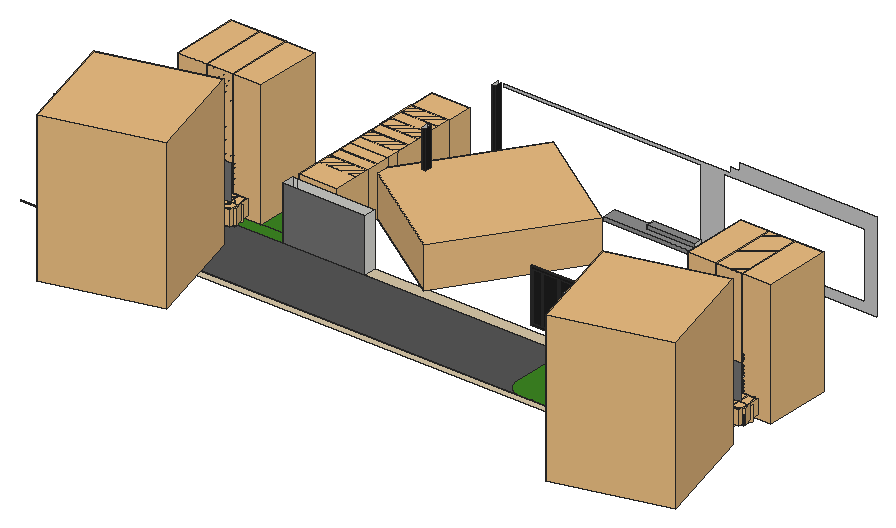
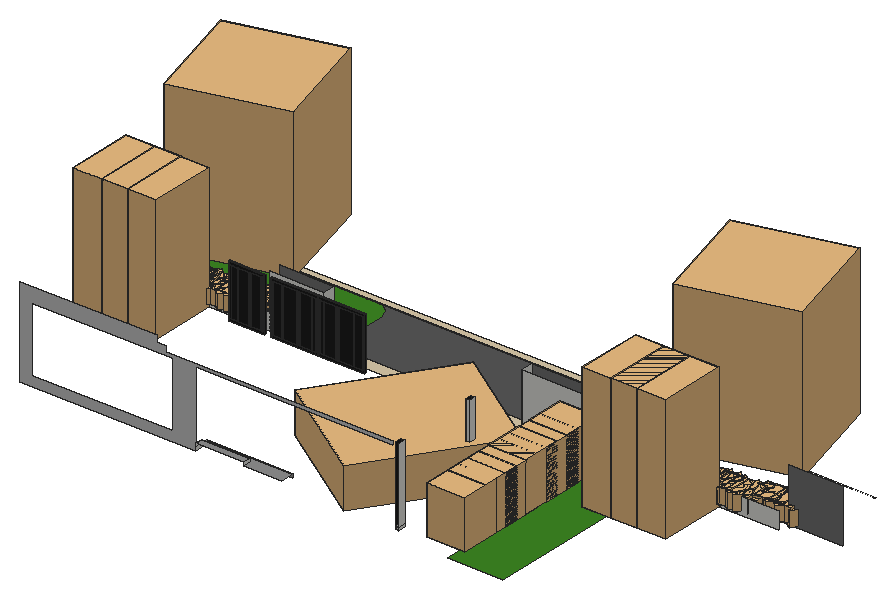
# SketchUp Ruby script. Lengths in inches.
U = 1.inch
M = Sketchup.active_model
def pt(a) = Geom::Point3d.new(a.map { |v| v * U })
def face(e, loops, mat)
  f = e.add_face(loops[0].map { |a| pt(a) })
  loops[1..].each { |l| e.add_face(l.map { |a| pt(a) }).erase! }
  f.material = f.back_material = mat if mat
  f
end
# faces: each face lists its corners as indices into pts; further lists are holes
def faces(e, pts, list, mat = nil) = list.each { |f| face(e, (f[0].is_a?(Array) ? f : [f]).map { |l| l.map { |i| pts[i] } }, mat) }
# xy, xz, yz: faces in a plane at the given z, y or x. An outline is a flat list of corners, or four numbers for a rectangle; further outlines are holes
def ring(l) = l.size == 4 ? [[l[0], l[1]], [l[2], l[1]], [l[2], l[3]], [l[0], l[3]]] : l.each_slice(2).to_a
def flat(e, list, mat, &to3) = list.each { |f| face(e, (f[0].is_a?(Array) ? f : [f]).map { |l| ring(l).map { |u, v| to3.(u, v) } }, mat) }
def xy(e, z, list, mat = nil) = flat(e, list, mat) { |x, y| [x, y, z] }
def xz(e, y, list, mat = nil) = flat(e, list, mat) { |x, z| [x, y, z] }
def yz(e, x, list, mat = nil) = flat(e, list, mat) { |y, z| [x, y, z] }
def lines(e, pts, list) = list.each { |a, b| e.add_line(pt(pts[a]), pt(pts[b])) }
# prism: a flat outline (further loops are holes) pulled along v
def prism(e, loops, v, mat = nil)
  f = face(e, loops, mat); d = Geom::Vector3d.new(v.map { |x| x * U })
  f.pushpull(f.normal.samedirection?(d) ? d.length : -d.length)
end
def box(e, o, s, mat = nil) = prism(e, [[o, [o[0] + s[0], o[1], o[2]], [o[0] + s[0], o[1] + s[1], o[2]], [o[0], o[1] + s[1], o[2]]]], [0, 0, s[2]], mat)
def at(x, y, z, deg = 0) = Geom::Transformation.translation(pt([x, y, z])) * Geom::Transformation.rotation(ORIGIN, Z_AXIS, deg.degrees)
def axes(o, x, y, z) = Geom::Transformation.new([*x, 0, *y, 0, *z, 0, *pt(o).to_a, 1])
def part(name) = M.definitions.add(name)
# library, detail: a bought-in or finely detailed component or shape, given as its bounding box
def library(name, o, s) = part(name).tap { |d| box(d.entities, o, s) }
def detail(e, o, s) = box(e.add_group.entities, o, s)
def put(e, d, t, mat = nil) = e.add_instance(d, t).tap { |i| i.material = mat if mat }
def group(e, t, mat = nil) = e.add_group.tap { |g| g.transformation = t; g.material = mat if mat }.entities
root = M.entities
M.materials.add("[Color M02]").color = [198, 198, 198]
M.materials.add("[Color M04]").color = [60, 133, 34]
M.materials.add("[Color M04]1").color = [142, 142, 142]
M.materials.add("[Color M05]1").color = [114, 114, 114]
M.materials.add("[Color M08]").color = [30, 30, 30]
M.materials.add("[Color_F16]").color = [51, 102, 0]
M.materials.add("[Field Square Tile]").color = [217, 201, 169]
M.materials.add("[Slate Light Tile]").color = [86, 86, 86]
c1 = library("Obj_000004",[-25.54,-25.36,-14.31],[50.67,50.64,41.42])
c2 = library("Obj_000003",[-31,-31.06,-7.89],[62,62.12,39.58])
c3 = library("Potted plant",[-29.7,0,-10.87],[31.67,38.52,72.45])
c4 = library("Palm tree",[-4.09,-4.52,0],[193.52,193.51,258.93])
c5 = part("Palm+Tree")
put(c5.entities,c4,at(25.51,-21.81,0,15))
c6 = library("plant (1)",[-35.72,-28.42,0],[66.31,67.39,84.38])
c7 = library("002+Bmw+M4+++mat3.4+2017",[-252.8,19.48,9.01],[196.94,171.32,55.15])
c8 = part("Group\#102")
g1 = group(c8.entities,at(0,0,0))
prism(g1,[[[0,3,72],[70.5,3,72],[70.5,3,0],[0,3,0]],[[67.5,3,3],[67.5,3,69],[3,3,69],[3,3,3]]],[0,-3,0])
c9 = part("Group\#135")
box(c9.entities,[0,0,0],[0.5,1,66])
c10 = part("Group\#148")
box(c10.entities,[0,-1,0],[5.5,1,66])
box(c10.entities,[50.84,-1,0],[13.66,1,66])
box(c10.entities,[28.06,-1,0],[22.28,1,66])
box(c10.entities,[24.66,-1,0],[2.9,1,66])
box(c10.entities,[6,-1,0],[18.16,1,66])
c11 = part("Component\#23")
g2 = group(c11.entities,at(70.5,0,0),"[Color M08]")
put(g2,c8,axes([70.5,0,0],[-1,0,0],[0,1,0],[0,0,1]))
g3 = group(g2,at(3,2,3))
g4 = group(g3,at(0,-1,0))
box(g4,[0,0,0],[5.5,1,66])
box(g4,[50.84,0,0],[13.66,1,66])
box(g4,[28.06,0,0],[22.28,1,66])
box(g4,[24.66,0,0],[2.9,1,66])
box(g4,[6,0,0],[18.16,1,66])
put(g3,c9,axes([50.34,0,0],[1,0,0],[0,-1,0],[0,0,1]))
put(g3,c9,axes([24.16,0,0],[1,0,0],[0,-1,0],[0,0,1]))
put(g3,c9,axes([27.56,0,0],[1,0,0],[0,-1,0],[0,0,1]))
put(g3,c9,axes([5.5,0,0],[1,0,0],[0,-1,0],[0,0,1]))
g5 = group(c11.entities,at(70.5,0,0),"[Color M08]")
put(g5,c8,at(-70.5,0,0))
g6 = group(g5,at(-3,2,3,-180))
put(g6,c10,at(0,1,0))
put(g6,c9,at(50.34,0,0))
put(g6,c9,at(24.16,0,0))
put(g6,c9,at(27.56,0,0))
put(g6,c9,at(5.5,0,0))
g7 = group(c11.entities,at(150,0,0),"[Color M08]")
put(g7,c8,axes([54,0,0],[-0.76596,0,0],[0,1,0],[0,0,1]))
g8 = group(g7,at(2.3,2,3))
put(g8,c10,axes([0,-1,0],[0.76596,0,0],[0,-1,0],[0,0,1]))
put(g8,c9,axes([38.55,0,0],[0.76596,0,0],[0,-1,0],[0,0,1]))
put(g8,c9,axes([18.5,0,0],[0.76596,0,0],[0,-1,0],[0,0,1]))
put(g8,c9,axes([21.11,0,0],[0.76596,0,0],[0,-1,0],[0,0,1]))
put(g8,c9,axes([4.22,0,0],[0.76596,0,0],[0,-1,0],[0,0,1]))
xy(root,-19.75,[[2463.16,10.6,2468.26,11.14,2473.25,12.39,2450.82,12.39,2452.96,11.68,2458.02,10.78],[1636.34,12.09,1641.55,12.39,1629.85,12.39,1631.12,12.24],[2522.8,12.09,2528.01,12.39,2516.3125,12.39,2517.58,12.24],[1938.63,143.39,1946.07,164.82],[1946.07,143.39,2081.32,164.82],
  [2037.07,322.71,2043.8,334.4375],[2037.07,475.3125,2043.8,487.3125]])
xy(root,-19.75,[[1841.83,12.39,1848.92,143.39],[2450.82,12.39,2735.38,12.39,2735.38,143.39,2426.02,143.39,2426.02,39.89,2427.39,34.93,2429.45,30.23,2432.14,25.85,2435.42,21.9,2439.22,18.4375,2443.47,15.55,2448.08,13.28],[1841.83,143.39,1938.63,164.82],[1841.83,164.82,1938.63,505.3125]],"[Color M04]")
xy(root,-19.75,[[2081.32,143.39,2426.02,164.82]],"[Field Square Tile]")
xy(root,-19.75,[[1848.92,12.39,2450.82,12.39,2448.08,13.28,2443.47,15.55,2439.22,18.4375,2435.42,21.9,2432.14,25.85,2429.45,30.23,2427.39,34.93,2426.02,39.89,2426.02,143.39,1848.92,143.39]],"[Slate Light Tile]")
xy(root,-19.3125,[[1841.83,0,1848.92,12.39],[1848.92,0,2735.38,12.39]],"[Field Square Tile]")
xy(root,-14.01,[[2240.94,464.0625,2391.36,464.0625,2391.36,474.5625,2306.98,474.5625,2306.98,487.3125,2240.94,487.3125]],"[Color M04]1")
xy(root,-8.01,[[2306.98,474.5625,2391.36,487.3125]],"[Color M04]1")
xz(root,12.39,[[1586.78,-19.75,1841.83,-19.3125],[1841.83,-19.75,1848.92,-19.3125],[1848.92,-19.75,2473.25,-19.3125],[2473.25,-19.75,2735.38,-19.3125]])
xz(root,143.39,[[1539.55,-19.75,1848.92,-19.75,1848.92,73,1787.65,73,1787.65,9.9375,1634.02,9.9375,1634.02,73,1539.55,73],[1938.63,-19.75,2081.32,73],[2426.02,-19.75,2735.38,-19.75,2735.38,73,2674.11,73,2674.11,9.9375,2520.48,9.9375,2520.48,73,2426.02,73]],"[Color M05]1")
xz(root,164.82,[[1634.02,-19.75,1787.65,9.9375],[1787.65,-19.75,1838.4,73],[1938.63,-19.75,1946.07,73],[1946.07,-19.75,1946.07,73,2081.32,73,2081.32,-19.75,2047.51,-19.75,2047.51,-15.625,2033.69,-15.625,2033.69,-19.75],[2033.69,-19.75,2047.51,-15.625],
  [2426.02,-19.75,2520.48,73],[2520.48,-19.75,2674.11,9.9375],[2674.11,-19.75,2724.86,73]])
xz(root,322.71,[[2037.07,-19.75,2043.8,-15.625]])
xz(root,322.71,[[2037.07,-15.625,2043.8,115.91]],"[Color M08]")
xz(root,334.4375,[[2037.07,-19.75,2043.8,-15.625],[2037.07,-15.625,2043.8,115.91]])
xz(root,464.0625,[[2240.94,-19.75,2391.36,-14.01]],"[Color M04]1")
xz(root,474.5625,[[2306.98,-14.01,2391.36,-8.01]],"[Color M04]1")
xz(root,475.3125,[[2037.07,-19.75,2043.8,-15.625]])
xz(root,475.3125,[[2037.07,-15.625,2043.8,115.91]],"[Color M08]")
xz(root,487.3125,[[2037.07,-19.75,2043.8,-15.625]])
xz(root,487.3125,[[[2391.36,-19.75,2696.7,-19.75,2696.7,136.125,2459.77,136.125,2459.77,125.0625,2444.15,125.0625,2444.15,123.92,2443.83,123.92,2443.83,117.06,2444.15,117.06,2444.15,115.91,2048.29,115.91,2048.29,110.1875,2391.36,110.1875],[2431.15,-3.75,2676.91,110.1875]]],"[Color M02]")
yz(root,1938.63,[[143.39,-19.75,164.82,73]])
yz(root,2037.07,[[322.71,-19.75,334.4375,-15.625],[475.3125,-19.75,487.3125,-15.625],[322.71,-15.625,334.4375,115.66],[475.3125,-15.625,487.3125,115.66]])
yz(root,2043.8,[[322.71,-19.75,334.4375,-15.625],[475.3125,-19.75,487.3125,-15.625]])
yz(root,2043.8,[[322.71,-15.625,334.4375,115.91],[475.3125,-15.625,487.3125,115.91]],"[Color M08]")
yz(root,2081.32,[[143.39,-19.75,164.82,73]])
yz(root,2306.98,[[474.5625,-14.01,487.3125,-8.01]])
yz(root,2391.36,[[464.0625,-19.75,487.3125,-14.01],[474.5625,-14.01,487.3125,-8.01]])
yz(root,2426.02,[[143.39,-19.75,164.82,73]])
put(root,c1,axes([1630.46,131.13,-8.96],[-0.54627,0.33345,-0.00035],[-0.33345,-0.54627,0.00015],[-0.00023,0.00031,0.64]))
put(root,c1,axes([1645.97,130.26,-8.96],[0.64,0,0],[0,0.64,0],[0,0,0.64]))
put(root,c2,axes([1645.97,130.26,-8.96],[0.64,0,0],[0,0.64,0],[0,0,0.64]),"[Color_F16]")
put(root,c1,axes([1646.38,130.18,-8.96],[0.45255,0.45255,-0.00035],[-0.45255,0.45255,0.00015],[0.00035,0.00015,0.64]))
put(root,c2,axes([1646.38,130.18,-8.96],[0.45255,0.45255,-0.00035],[-0.45255,0.45255,0.00015],[0.00035,0.00015,0.64]),"[Color_F16]")
put(root,c1,axes([1661.85,130.26,-8.96],[0.64,0,0],[0,0.64,0],[0,0,0.64]))
put(root,c2,axes([1661.85,130.26,-8.96],[0.64,0,0],[0,0.64,0],[0,0,0.64]),"[Color_F16]")
put(root,c1,axes([1662.26,130.18,-8.96],[0.45255,0.45255,-0.00035],[-0.45255,0.45255,0.00015],[0.00035,0.00015,0.64]))
put(root,c2,axes([1662.26,130.18,-8.96],[0.45255,0.45255,-0.00035],[-0.45255,0.45255,0.00015],[0.00035,0.00015,0.64]),"[Color_F16]")
put(root,c1,axes([1677.44,130.52,-8.96],[0.28256,0.57425,0],[-0.57425,0.28256,0],[0,0,0.64]))
put(root,c2,axes([1677.69,130.86,-8.96],[-0.20625,0.60586,-0.00035],[-0.60586,-0.20625,0.00015],[0.00002,0.00038,0.64]),"[Color_F16]")
put(root,c2,axes([1677.72,130.26,-8.96],[0.64,0,0],[0,0.64,0],[0,0,0.64]),"[Color_F16]")
put(root,c1,axes([1677.69,130.86,-8.96],[-0.20625,0.60586,-0.00035],[-0.60586,-0.20625,0.00015],[0.00002,0.00038,0.64]))
put(root,c1,axes([1692.19,144.21,-8.16],[0.64,0,0],[0,0.64,0],[0,0,0.64]))
put(root,c1,axes([1708.0625,144.21,-8.16],[0.64,0,0],[0,0.64,0],[0,0,0.64]))
put(root,c2,axes([1708.0625,144.21,-8.16],[0.64,0,0],[0,0.64,0],[0,0,0.64]),"[Color_F16]")
put(root,c1,axes([1708.47,144.13,-8.16],[0.45255,0.45255,-0.00035],[-0.45255,0.45255,0.00015],[0.00035,0.00015,0.64]))
put(root,c2,axes([1708.47,144.13,-8.16],[0.45255,0.45255,-0.00035],[-0.45255,0.45255,0.00015],[0.00035,0.00015,0.64]),"[Color_F16]")
put(root,c2,axes([1724.3,145.08,-8.16],[-0.54627,0.33345,-0.00035],[-0.33345,-0.54627,0.00015],[-0.00023,0.00031,0.64]),"[Color_F16]")
put(root,c2,axes([1724.32,144.66,-8.16],[-0.15049,0.62206,0],[-0.62206,-0.15049,0],[0,0,0.64]),"[Color_F16]")
put(root,c1,axes([1724.32,144.66,-8.16],[-0.15049,0.62206,0],[-0.62206,-0.15049,0],[0,0,0.64]))
put(root,c1,axes([1724.3,145.08,-8.16],[-0.54627,0.33345,-0.00035],[-0.33345,-0.54627,0.00015],[-0.00023,0.00031,0.64]))
put(root,c1,axes([1739.8125,144.21,-8.16],[0.64,0,0],[0,0.64,0],[0,0,0.64]))
put(root,c2,axes([1739.8125,144.21,-8.16],[0.64,0,0],[0,0.64,0],[0,0,0.64]),"[Color_F16]")
put(root,c1,axes([1740.22,144.13,-8.16],[0.45255,0.45255,-0.00035],[-0.45255,0.45255,0.00015],[0.00035,0.00015,0.64]))
put(root,c2,axes([1740.22,144.13,-8.16],[0.45255,0.45255,-0.00035],[-0.45255,0.45255,0.00015],[0.00035,0.00015,0.64]),"[Color_F16]")
put(root,c1,axes([1755.6875,144.21,-8.16],[0.64,0,0],[0,0.64,0],[0,0,0.64]))
put(root,c2,axes([1755.6875,144.21,-8.16],[0.64,0,0],[0,0.64,0],[0,0,0.64]),"[Color_F16]")
put(root,c1,axes([1756.1,144.13,-8.16],[0.45255,0.45255,-0.00035],[-0.45255,0.45255,0.00015],[0.00035,0.00015,0.64]))
put(root,c2,axes([1756.1,144.13,-8.16],[0.45255,0.45255,-0.00035],[-0.45255,0.45255,0.00015],[0.00035,0.00015,0.64]),"[Color_F16]")
put(root,c1,axes([1762.56,144.21,-8.16],[0.64,0,0],[0,0.64,0],[0,0,0.64]))
put(root,c1,axes([1771.27,144.47,-8.16],[0.28256,0.57425,0],[-0.57425,0.28256,0],[0,0,0.64]))
put(root,c2,axes([1771.52,144.81,-8.16],[-0.20625,0.60586,-0.00035],[-0.60586,-0.20625,0.00015],[0.00002,0.00038,0.64]),"[Color_F16]")
put(root,c2,axes([1771.56,144.21,-8.16],[0.64,0,0],[0,0.64,0],[0,0,0.64]),"[Color_F16]")
put(root,c1,axes([1771.52,144.81,-8.16],[-0.20625,0.60586,-0.00035],[-0.60586,-0.20625,0.00015],[0.00002,0.00038,0.64]))
put(root,c1,axes([1778.4375,144.21,-8.16],[0.64,0,0],[0,0.64,0],[0,0,0.64]))
put(root,c2,axes([1778.4375,144.21,-8.16],[0.64,0,0],[0,0.64,0],[0,0,0.64]),"[Color_F16]")
put(root,c1,axes([1778.85,144.13,-8.16],[0.45255,0.45255,-0.00035],[-0.45255,0.45255,0.00015],[0.00035,0.00015,0.64]))
put(root,c2,axes([1778.85,144.13,-8.16],[0.45255,0.45255,-0.00035],[-0.45255,0.45255,0.00015],[0.00035,0.00015,0.64]),"[Color_F16]")
put(root,c3,axes([1828.5,164.82,12.86],[3,0,0],[0,3,0],[0,0,3]))
put(root,c2,axes([1794.68,145.08,-8.16],[-0.54627,0.33345,-0.00035],[-0.33345,-0.54627,0.00015],[-0.00023,0.00031,0.64]),"[Color_F16]")
put(root,c2,axes([1794.7,144.66,-8.16],[-0.15049,0.62206,0],[-0.62206,-0.15049,0],[0,0,0.64]),"[Color_F16]")
put(root,c1,axes([1794.7,144.66,-8.16],[-0.15049,0.62206,0],[-0.62206,-0.15049,0],[0,0,0.64]))
put(root,c1,axes([1794.68,145.08,-8.16],[-0.54627,0.33345,-0.00035],[-0.33345,-0.54627,0.00015],[-0.00023,0.00031,0.64]))
put(root,c1,axes([1810.1875,144.21,-8.16],[0.64,0,0],[0,0.64,0],[0,0,0.64]))
put(root,c2,axes([1810.1875,144.21,-8.16],[0.64,0,0],[0,0.64,0],[0,0,0.64]),"[Color_F16]")
put(root,c1,axes([1810.6,144.13,-8.16],[0.45255,0.45255,-0.00035],[-0.45255,0.45255,0.00015],[0.00035,0.00015,0.64]))
put(root,c2,axes([1810.6,144.13,-8.16],[0.45255,0.45255,-0.00035],[-0.45255,0.45255,0.00015],[0.00035,0.00015,0.64]),"[Color_F16]")
put(root,c5,at(1723.85,-125.125,-17.22))
put(root,c1,axes([1826.0625,144.21,-8.16],[0.64,0,0],[0,0.64,0],[0,0,0.64]))
put(root,c2,axes([1826.0625,144.21,-8.16],[0.64,0,0],[0,0.64,0],[0,0,0.64]),"[Color_F16]")
put(root,c1,axes([1826.47,144.13,-8.16],[0.45255,0.45255,-0.00035],[-0.45255,0.45255,0.00015],[0.00035,0.00015,0.64]))
put(root,c2,axes([1826.47,144.13,-8.16],[0.45255,0.45255,-0.00035],[-0.45255,0.45255,0.00015],[0.00035,0.00015,0.64]),"[Color_F16]")
put(root,c3,axes([1878.375,164.82,12.86],[3,0,0],[0,3,0],[0,0,3]))
put(root,c1,axes([1841.65,144.47,-8.16],[0.28256,0.57425,0],[-0.57425,0.28256,0],[0,0,0.64]))
put(root,c2,axes([1841.9,144.81,-8.16],[-0.20625,0.60586,-0.00035],[-0.60586,-0.20625,0.00015],[0.00002,0.00038,0.64]),"[Color_F16]")
put(root,c2,axes([1841.93,144.21,-8.16],[0.64,0,0],[0,0.64,0],[0,0,0.64]),"[Color_F16]")
put(root,c1,axes([1841.9,144.81,-8.16],[-0.20625,0.60586,-0.00035],[-0.60586,-0.20625,0.00015],[0.00002,0.00038,0.64]))
put(root,c6,at(1966.18,216.8,-19.75))
put(root,c6,at(1966.18,261.11,-19.75))
put(root,c6,at(1966.18,305.42,-19.75))
put(root,c6,at(1966.18,349.73,-19.75))
put(root,c6,at(1966.18,394.05,-19.75))
put(root,c6,at(1966.18,438.36,-19.75))
put(root,c7,axes([2374.11,415.92,-31.37],[0.71831,1.07151,0],[-1.07151,0.71831,0],[0,0,1.29]))
put(root,c11,axes([2344.87,175.05,-19.75],[1.16,0,0],[0,1.16,0],[0,0,1.28819]))
put(root,c1,axes([2484.82,130.26,-8.96],[0.64,0,0],[0,0.64,0],[0,0,0.64]))
put(root,c1,axes([2500.69,130.26,-8.96],[0.64,0,0],[0,0.64,0],[0,0,0.64]))
put(root,c2,axes([2500.69,130.26,-8.96],[0.64,0,0],[0,0.64,0],[0,0,0.64]),"[Color_F16]")
put(root,c1,axes([2501.1,130.18,-8.96],[0.45255,0.45255,-0.00035],[-0.45255,0.45255,0.00015],[0.00035,0.00015,0.64]))
put(root,c2,axes([2501.1,130.18,-8.96],[0.45255,0.45255,-0.00035],[-0.45255,0.45255,0.00015],[0.00035,0.00015,0.64]),"[Color_F16]")
put(root,c2,axes([2516.93,131.13,-8.96],[-0.54627,0.33345,-0.00035],[-0.33345,-0.54627,0.00015],[-0.00023,0.00031,0.64]),"[Color_F16]")
put(root,c2,axes([2516.95,130.71,-8.96],[-0.15049,0.62206,0],[-0.62206,-0.15049,0],[0,0,0.64]),"[Color_F16]")
put(root,c1,axes([2516.95,130.71,-8.96],[-0.15049,0.62206,0],[-0.62206,-0.15049,0],[0,0,0.64]))
put(root,c1,axes([2516.93,131.13,-8.96],[-0.54627,0.33345,-0.00035],[-0.33345,-0.54627,0.00015],[-0.00023,0.00031,0.64]))
put(root,c1,axes([2532.4375,130.26,-8.96],[0.64,0,0],[0,0.64,0],[0,0,0.64]))
put(root,c2,axes([2532.4375,130.26,-8.96],[0.64,0,0],[0,0.64,0],[0,0,0.64]),"[Color_F16]")
put(root,c1,axes([2532.85,130.18,-8.96],[0.45255,0.45255,-0.00035],[-0.45255,0.45255,0.00015],[0.00035,0.00015,0.64]))
put(root,c2,axes([2532.85,130.18,-8.96],[0.45255,0.45255,-0.00035],[-0.45255,0.45255,0.00015],[0.00035,0.00015,0.64]),"[Color_F16]")
put(root,c1,axes([2548.3125,130.26,-8.96],[0.64,0,0],[0,0.64,0],[0,0,0.64]))
put(root,c2,axes([2548.3125,130.26,-8.96],[0.64,0,0],[0,0.64,0],[0,0,0.64]),"[Color_F16]")
put(root,c1,axes([2548.72,130.18,-8.96],[0.45255,0.45255,-0.00035],[-0.45255,0.45255,0.00015],[0.00035,0.00015,0.64]))
put(root,c2,axes([2548.72,130.18,-8.96],[0.45255,0.45255,-0.00035],[-0.45255,0.45255,0.00015],[0.00035,0.00015,0.64]),"[Color_F16]")
put(root,c1,axes([2563.9,130.52,-8.96],[0.28256,0.57425,0],[-0.57425,0.28256,0],[0,0,0.64]))
put(root,c2,axes([2564.15,130.86,-8.96],[-0.20625,0.60586,-0.00035],[-0.60586,-0.20625,0.00015],[0.00002,0.00038,0.64]),"[Color_F16]")
put(root,c2,axes([2564.1875,130.26,-8.96],[0.64,0,0],[0,0.64,0],[0,0,0.64]),"[Color_F16]")
put(root,c1,axes([2564.15,130.86,-8.96],[-0.20625,0.60586,-0.00035],[-0.60586,-0.20625,0.00015],[0.00002,0.00038,0.64]))
put(root,c1,axes([2578.65,144.21,-8.16],[0.64,0,0],[0,0.64,0],[0,0,0.64]))
put(root,c1,axes([2594.53,144.21,-8.16],[0.64,0,0],[0,0.64,0],[0,0,0.64]))
put(root,c2,axes([2594.53,144.21,-8.16],[0.64,0,0],[0,0.64,0],[0,0,0.64]),"[Color_F16]")
put(root,c1,axes([2594.9375,144.13,-8.16],[0.45255,0.45255,-0.00035],[-0.45255,0.45255,0.00015],[0.00035,0.00015,0.64]))
put(root,c2,axes([2594.9375,144.13,-8.16],[0.45255,0.45255,-0.00035],[-0.45255,0.45255,0.00015],[0.00035,0.00015,0.64]),"[Color_F16]")
put(root,c2,axes([2610.76,145.08,-8.16],[-0.54627,0.33345,-0.00035],[-0.33345,-0.54627,0.00015],[-0.00023,0.00031,0.64]),"[Color_F16]")
put(root,c2,axes([2610.79,144.66,-8.16],[-0.15049,0.62206,0],[-0.62206,-0.15049,0],[0,0,0.64]),"[Color_F16]")
put(root,c1,axes([2610.79,144.66,-8.16],[-0.15049,0.62206,0],[-0.62206,-0.15049,0],[0,0,0.64]))
put(root,c1,axes([2610.76,145.08,-8.16],[-0.54627,0.33345,-0.00035],[-0.33345,-0.54627,0.00015],[-0.00023,0.00031,0.64]))
put(root,c1,axes([2626.28,144.21,-8.16],[0.64,0,0],[0,0.64,0],[0,0,0.64]))
put(root,c2,axes([2626.28,144.21,-8.16],[0.64,0,0],[0,0.64,0],[0,0,0.64]),"[Color_F16]")
put(root,c1,axes([2626.69,144.13,-8.16],[0.45255,0.45255,-0.00035],[-0.45255,0.45255,0.00015],[0.00035,0.00015,0.64]))
put(root,c2,axes([2626.69,144.13,-8.16],[0.45255,0.45255,-0.00035],[-0.45255,0.45255,0.00015],[0.00035,0.00015,0.64]),"[Color_F16]")
put(root,c1,axes([2642.15,144.21,-8.16],[0.64,0,0],[0,0.64,0],[0,0,0.64]))
put(root,c2,axes([2642.15,144.21,-8.16],[0.64,0,0],[0,0.64,0],[0,0,0.64]),"[Color_F16]")
put(root,c1,axes([2642.56,144.13,-8.16],[0.45255,0.45255,-0.00035],[-0.45255,0.45255,0.00015],[0.00035,0.00015,0.64]))
put(root,c2,axes([2642.56,144.13,-8.16],[0.45255,0.45255,-0.00035],[-0.45255,0.45255,0.00015],[0.00035,0.00015,0.64]),"[Color_F16]")
put(root,c1,axes([2649.03,144.21,-8.16],[0.64,0,0],[0,0.64,0],[0,0,0.64]))
put(root,c1,axes([2657.74,144.47,-8.16],[0.28256,0.57425,0],[-0.57425,0.28256,0],[0,0,0.64]))
put(root,c2,axes([2657.99,144.81,-8.16],[-0.20625,0.60586,-0.00035],[-0.60586,-0.20625,0.00015],[0.00002,0.00038,0.64]),"[Color_F16]")
put(root,c2,axes([2658.02,144.21,-8.16],[0.64,0,0],[0,0.64,0],[0,0,0.64]),"[Color_F16]")
put(root,c1,axes([2657.99,144.81,-8.16],[-0.20625,0.60586,-0.00035],[-0.60586,-0.20625,0.00015],[0.00002,0.00038,0.64]))
put(root,c1,axes([2664.9,144.21,-8.16],[0.64,0,0],[0,0.64,0],[0,0,0.64]))
put(root,c2,axes([2664.9,144.21,-8.16],[0.64,0,0],[0,0.64,0],[0,0,0.64]),"[Color_F16]")
put(root,c1,axes([2665.3125,144.13,-8.16],[0.45255,0.45255,-0.00035],[-0.45255,0.45255,0.00015],[0.00035,0.00015,0.64]))
put(root,c2,axes([2665.3125,144.13,-8.16],[0.45255,0.45255,-0.00035],[-0.45255,0.45255,0.00015],[0.00035,0.00015,0.64]),"[Color_F16]")
put(root,c3,axes([2714.96,164.82,12.86],[3,0,0],[0,3,0],[0,0,3]))
put(root,c2,axes([2681.14,145.08,-8.16],[-0.54627,0.33345,-0.00035],[-0.33345,-0.54627,0.00015],[-0.00023,0.00031,0.64]),"[Color_F16]")
put(root,c2,axes([2681.16,144.66,-8.16],[-0.15049,0.62206,0],[-0.62206,-0.15049,0],[0,0,0.64]),"[Color_F16]")
put(root,c1,axes([2681.16,144.66,-8.16],[-0.15049,0.62206,0],[-0.62206,-0.15049,0],[0,0,0.64]))
put(root,c1,axes([2681.14,145.08,-8.16],[-0.54627,0.33345,-0.00035],[-0.33345,-0.54627,0.00015],[-0.00023,0.00031,0.64]))
put(root,c1,axes([2696.65,144.21,-8.16],[0.64,0,0],[0,0.64,0],[0,0,0.64]))
put(root,c2,axes([2696.65,144.21,-8.16],[0.64,0,0],[0,0.64,0],[0,0,0.64]),"[Color_F16]")
put(root,c1,axes([2697.06,144.13,-8.16],[0.45255,0.45255,-0.00035],[-0.45255,0.45255,0.00015],[0.00035,0.00015,0.64]))
put(root,c2,axes([2697.06,144.13,-8.16],[0.45255,0.45255,-0.00035],[-0.45255,0.45255,0.00015],[0.00035,0.00015,0.64]),"[Color_F16]")
put(root,c5,at(2610.3125,-125.125,-17.22))
put(root,c1,axes([2712.52,144.21,-8.16],[0.64,0,0],[0,0.64,0],[0,0,0.64]))
put(root,c2,axes([2712.52,144.21,-8.16],[0.64,0,0],[0,0.64,0],[0,0,0.64]),"[Color_F16]")
put(root,c1,axes([2712.93,144.13,-8.16],[0.45255,0.45255,-0.00035],[-0.45255,0.45255,0.00015],[0.00035,0.00015,0.64]))
put(root,c2,axes([2712.93,144.13,-8.16],[0.45255,0.45255,-0.00035],[-0.45255,0.45255,0.00015],[0.00035,0.00015,0.64]),"[Color_F16]")
put(root,c3,axes([2764.84,164.82,12.86],[3,0,0],[0,3,0],[0,0,3]))
put(root,c1,axes([2728.11,144.47,-8.16],[0.28256,0.57425,0],[-0.57425,0.28256,0],[0,0,0.64]))
put(root,c2,axes([2728.36,144.81,-8.16],[-0.20625,0.60586,-0.00035],[-0.60586,-0.20625,0.00015],[0.00002,0.00038,0.64]),"[Color_F16]")
put(root,c2,axes([2728.4,144.21,-8.16],[0.64,0,0],[0,0.64,0],[0,0,0.64]),"[Color_F16]")
put(root,c1,axes([2728.36,144.81,-8.16],[-0.20625,0.60586,-0.00035],[-0.60586,-0.20625,0.00015],[0.00002,0.00038,0.64]))
